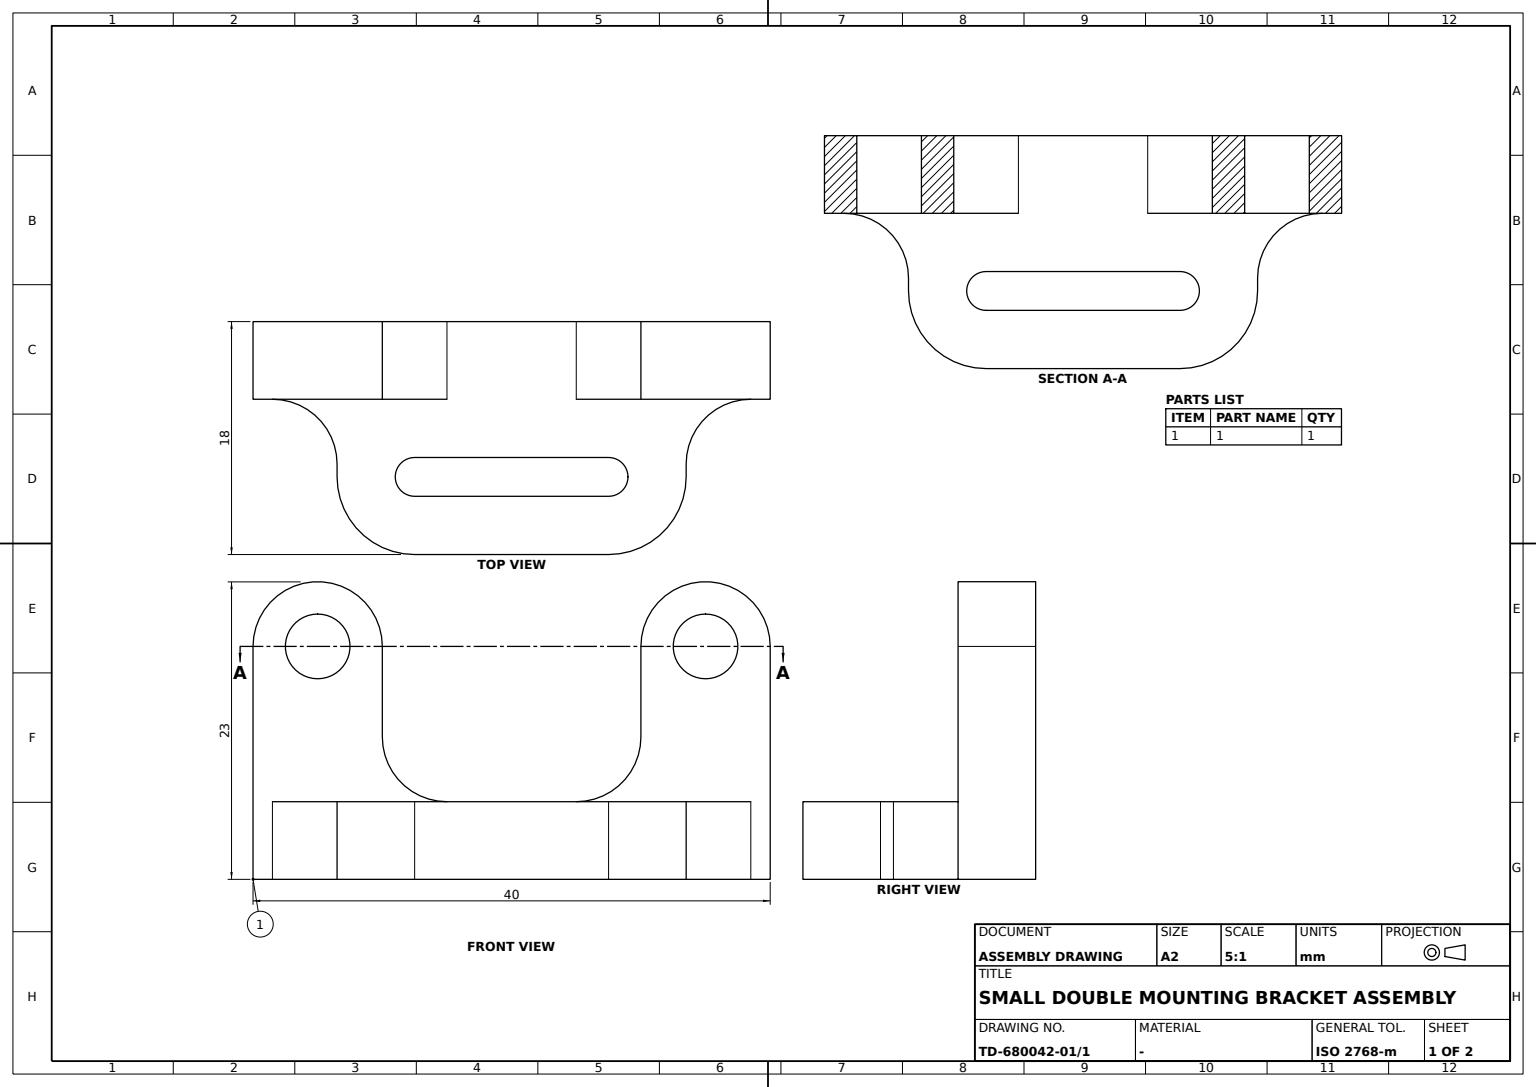
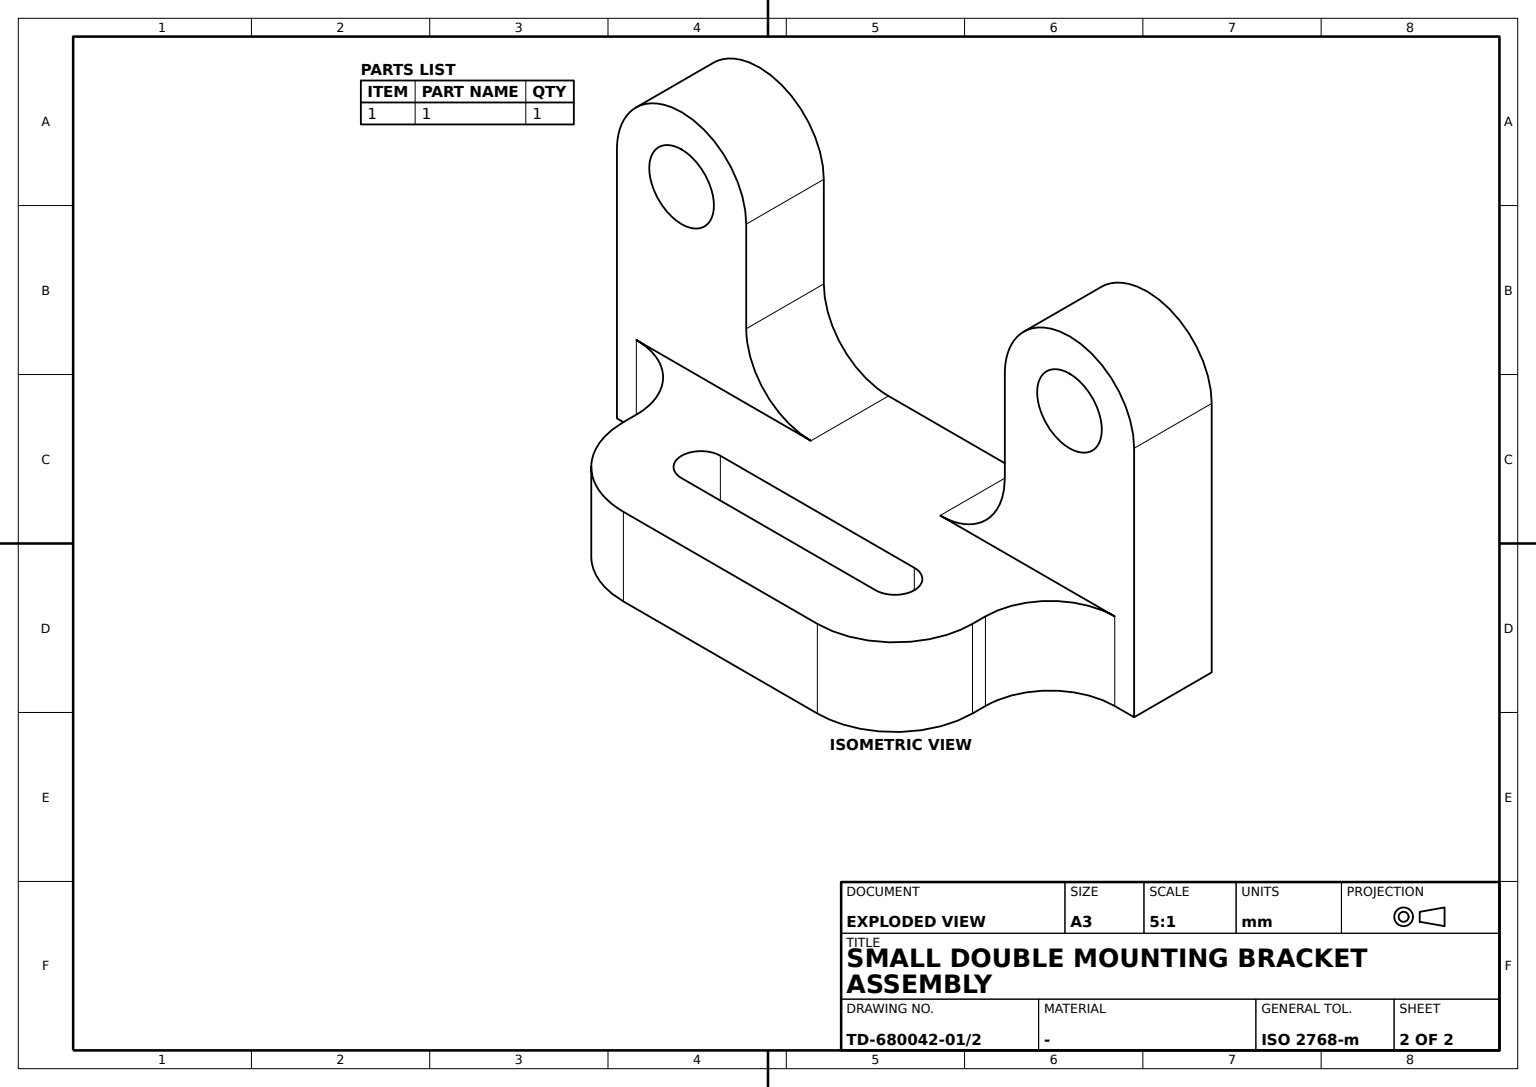
ISO-10303-21;
HEADER;
FILE_DESCRIPTION((''),'2;1');
FILE_NAME('','',(''),(''),'','','');
FILE_SCHEMA(('AUTOMOTIVE_DESIGN'));
ENDSEC;
DATA;
#1=APPLICATION_CONTEXT('');
#2=PRODUCT_CONTEXT('',#1,'mechanical');
#3=PRODUCT('','','',(#2));
#4=PRODUCT_DEFINITION_FORMATION('','',#3);
#5=PRODUCT_DEFINITION_CONTEXT('',#1,'design');
#6=PRODUCT_DEFINITION('','',#4,#5);
#7=PRODUCT_DEFINITION_SHAPE('','',#6);
#8=(LENGTH_UNIT()NAMED_UNIT(*)SI_UNIT(.MILLI.,.METRE.));
#9=(NAMED_UNIT(*)PLANE_ANGLE_UNIT()SI_UNIT($,.RADIAN.));
#10=(NAMED_UNIT(*)SI_UNIT($,.STERADIAN.)SOLID_ANGLE_UNIT());
#11=UNCERTAINTY_MEASURE_WITH_UNIT(LENGTH_MEASURE(1.E-05),#8,'distance_accuracy_value','');
#12=(GEOMETRIC_REPRESENTATION_CONTEXT(3)GLOBAL_UNCERTAINTY_ASSIGNED_CONTEXT((#11))GLOBAL_UNIT_ASSIGNED_CONTEXT((#8,#9,#10))REPRESENTATION_CONTEXT('',''));
#13=CARTESIAN_POINT('',(-5.,-6.,6.));
#14=VERTEX_POINT('',#13);
#15=CARTESIAN_POINT('',(-10.,-6.,11.));
#16=VERTEX_POINT('',#15);
#17=CARTESIAN_POINT('',(-5.,-6.,11.));
#18=DIRECTION('',(0.,1.,0.));
#19=DIRECTION('',(0.,0.,1.));
#20=AXIS2_PLACEMENT_3D('',#17,#18,#19);
#21=CIRCLE('',#20,5.);
#22=EDGE_CURVE('',#14,#16,#21,.T.);
#23=ORIENTED_EDGE('',*,*,#22,.T.);
#24=CARTESIAN_POINT('',(-10.,-6.,18.));
#25=VERTEX_POINT('',#24);
#26=DIRECTION('',(0.,0.,-1.));
#27=VECTOR('',#26,1000.);
#28=LINE('',#24,#27);
#29=EDGE_CURVE('',#25,#16,#28,.T.);
#30=ORIENTED_EDGE('',*,*,#29,.F.);
#31=CARTESIAN_POINT('',(-20.,-6.,18.));
#32=VERTEX_POINT('',#31);
#33=CARTESIAN_POINT('',(-15.,-6.,18.));
#34=DIRECTION('',(0.,-1.,0.));
#35=DIRECTION('',(1.,0.,0.));
#36=AXIS2_PLACEMENT_3D('',#33,#34,#35);
#37=CIRCLE('',#36,5.);
#38=EDGE_CURVE('',#25,#32,#37,.T.);
#39=ORIENTED_EDGE('',*,*,#38,.T.);
#40=CARTESIAN_POINT('',(-20.,-6.,0.));
#41=VERTEX_POINT('',#40);
#42=LINE('',#31,#27);
#43=EDGE_CURVE('',#32,#41,#42,.T.);
#44=ORIENTED_EDGE('',*,*,#43,.T.);
#45=CARTESIAN_POINT('',(-18.5,-6.,0.));
#46=VERTEX_POINT('',#45);
#47=CARTESIAN_POINT('',(-13.5,-6.,0.));
#48=DIRECTION('',(-1.,0.,0.));
#49=VECTOR('',#48,1000.);
#50=LINE('',#47,#49);
#51=EDGE_CURVE('',#46,#41,#50,.T.);
#52=ORIENTED_EDGE('',*,*,#51,.F.);
#53=CARTESIAN_POINT('',(-18.5,-6.,6.));
#54=VERTEX_POINT('',#53);
#55=VECTOR('',#19,1000.);
#56=LINE('',#53,#55);
#57=EDGE_CURVE('',#46,#54,#56,.T.);
#58=ORIENTED_EDGE('',*,*,#57,.T.);
#59=CARTESIAN_POINT('',(20.,-6.,6.));
#60=LINE('',#59,#49);
#61=EDGE_CURVE('',#14,#54,#60,.T.);
#62=ORIENTED_EDGE('',*,*,#61,.F.);
#63=EDGE_LOOP('',(#23,#30,#39,#44,#52,#58,#62));
#64=FACE_OUTER_BOUND('',#63,.T.);
#65=CARTESIAN_POINT('',(-15.,-6.,20.5));
#66=VERTEX_POINT('',#65);
#67=CARTESIAN_POINT('',(-15.,-6.,15.5));
#68=VERTEX_POINT('',#67);
#69=CIRCLE('',#36,2.5);
#70=EDGE_CURVE('',#66,#68,#69,.T.);
#71=ORIENTED_EDGE('',*,*,#70,.F.);
#72=EDGE_CURVE('',#68,#66,#69,.T.);
#73=ORIENTED_EDGE('',*,*,#72,.F.);
#74=EDGE_LOOP('',(#71,#73));
#75=FACE_BOUND('',#74,.T.);
#76=CARTESIAN_POINT('',(20.,-6.,18.));
#77=AXIS2_PLACEMENT_3D('',#76,#18,#19);
#78=PLANE('',#77);
#79=ADVANCED_FACE('',(#64,#75),#78,.F.);
#80=CARTESIAN_POINT('',(-13.5,-11.,6.));
#81=VERTEX_POINT('',#80);
#82=CARTESIAN_POINT('',(-18.5,-11.,6.));
#83=AXIS2_PLACEMENT_3D('',#82,#26,#48);
#84=CIRCLE('',#83,5.);
#85=EDGE_CURVE('',#54,#81,#84,.T.);
#86=ORIENTED_EDGE('',*,*,#85,.F.);
#87=ORIENTED_EDGE('',*,*,#57,.F.);
#88=CARTESIAN_POINT('',(-13.5,-11.,0.));
#89=VERTEX_POINT('',#88);
#90=CARTESIAN_POINT('',(-18.5,-11.,0.));
#91=AXIS2_PLACEMENT_3D('',#90,#19,#34);
#92=CIRCLE('',#91,5.);
#93=EDGE_CURVE('',#89,#46,#92,.T.);
#94=ORIENTED_EDGE('',*,*,#93,.F.);
#95=LINE('',#88,#27);
#96=EDGE_CURVE('',#81,#89,#95,.T.);
#97=ORIENTED_EDGE('',*,*,#96,.F.);
#98=EDGE_LOOP('',(#86,#87,#94,#97));
#99=FACE_OUTER_BOUND('',#98,.T.);
#100=CARTESIAN_POINT('',(-18.5,-11.,18.));
#101=AXIS2_PLACEMENT_3D('',#100,#26,#18);
#102=CYLINDRICAL_SURFACE('',#101,5.);
#103=ADVANCED_FACE('',(#99),#102,.F.);
#104=CARTESIAN_POINT('',(9.,-12.,0.));
#105=VERTEX_POINT('',#104);
#106=CARTESIAN_POINT('',(9.,-12.,6.));
#107=VERTEX_POINT('',#106);
#108=LINE('',#104,#55);
#109=EDGE_CURVE('',#105,#107,#108,.T.);
#110=ORIENTED_EDGE('',*,*,#109,.F.);
#111=CARTESIAN_POINT('',(7.5,-13.5,0.));
#112=VERTEX_POINT('',#111);
#113=CARTESIAN_POINT('',(7.5,-12.,0.));
#114=AXIS2_PLACEMENT_3D('',#113,#19,#35);
#115=CIRCLE('',#114,1.5);
#116=EDGE_CURVE('',#112,#105,#115,.T.);
#117=ORIENTED_EDGE('',*,*,#116,.F.);
#118=CARTESIAN_POINT('',(7.5,-13.5,6.));
#119=VERTEX_POINT('',#118);
#120=LINE('',#111,#27);
#121=EDGE_CURVE('',#119,#112,#120,.T.);
#122=ORIENTED_EDGE('',*,*,#121,.F.);
#123=CARTESIAN_POINT('',(7.5,-12.,6.));
#124=AXIS2_PLACEMENT_3D('',#123,#19,#35);
#125=CIRCLE('',#124,1.5);
#126=EDGE_CURVE('',#119,#107,#125,.T.);
#127=ORIENTED_EDGE('',*,*,#126,.T.);
#128=EDGE_LOOP('',(#110,#117,#122,#127));
#129=FACE_OUTER_BOUND('',#128,.T.);
#130=CYLINDRICAL_SURFACE('',#114,1.5);
#131=ADVANCED_FACE('',(#129),#130,.F.);
#132=CARTESIAN_POINT('',(10.,-6.,11.));
#133=VERTEX_POINT('',#132);
#134=CARTESIAN_POINT('',(5.,-6.,6.));
#135=VERTEX_POINT('',#134);
#136=CARTESIAN_POINT('',(5.,-6.,11.));
#137=AXIS2_PLACEMENT_3D('',#136,#18,#19);
#138=CIRCLE('',#137,5.);
#139=EDGE_CURVE('',#133,#135,#138,.T.);
#140=ORIENTED_EDGE('',*,*,#139,.F.);
#141=CARTESIAN_POINT('',(10.,0.,11.));
#142=VERTEX_POINT('',#141);
#143=VECTOR('',#34,1000.);
#144=LINE('',#132,#143);
#145=EDGE_CURVE('',#142,#133,#144,.T.);
#146=ORIENTED_EDGE('',*,*,#145,.F.);
#147=CARTESIAN_POINT('',(5.,0.,6.));
#148=VERTEX_POINT('',#147);
#149=CARTESIAN_POINT('',(5.,0.,11.));
#150=AXIS2_PLACEMENT_3D('',#149,#34,#26);
#151=CIRCLE('',#150,5.);
#152=EDGE_CURVE('',#148,#142,#151,.T.);
#153=ORIENTED_EDGE('',*,*,#152,.F.);
#154=VECTOR('',#18,1000.);
#155=LINE('',#147,#154);
#156=EDGE_CURVE('',#135,#148,#155,.T.);
#157=ORIENTED_EDGE('',*,*,#156,.F.);
#158=EDGE_LOOP('',(#140,#146,#153,#157));
#159=FACE_OUTER_BOUND('',#158,.T.);
#160=CARTESIAN_POINT('',(5.,34.,11.));
#161=AXIS2_PLACEMENT_3D('',#160,#18,#19);
#162=CYLINDRICAL_SURFACE('',#161,5.);
#163=ADVANCED_FACE('',(#159),#162,.F.);
#164=CARTESIAN_POINT('',(-7.5,-10.5,6.));
#165=VERTEX_POINT('',#164);
#166=CARTESIAN_POINT('',(-7.5,-13.5,6.));
#167=VERTEX_POINT('',#166);
#168=CARTESIAN_POINT('',(-7.5,-12.,6.));
#169=AXIS2_PLACEMENT_3D('',#168,#19,#35);
#170=CIRCLE('',#169,1.5);
#171=EDGE_CURVE('',#165,#167,#170,.T.);
#172=ORIENTED_EDGE('',*,*,#171,.T.);
#173=CARTESIAN_POINT('',(-7.5,-13.5,0.));
#174=VERTEX_POINT('',#173);
#175=LINE('',#173,#27);
#176=EDGE_CURVE('',#167,#174,#175,.T.);
#177=ORIENTED_EDGE('',*,*,#176,.T.);
#178=CARTESIAN_POINT('',(-7.5,-10.5,0.));
#179=VERTEX_POINT('',#178);
#180=CARTESIAN_POINT('',(-7.5,-12.,0.));
#181=AXIS2_PLACEMENT_3D('',#180,#19,#35);
#182=CIRCLE('',#181,1.5);
#183=EDGE_CURVE('',#179,#174,#182,.T.);
#184=ORIENTED_EDGE('',*,*,#183,.F.);
#185=LINE('',#178,#27);
#186=EDGE_CURVE('',#165,#179,#185,.T.);
#187=ORIENTED_EDGE('',*,*,#186,.F.);
#188=EDGE_LOOP('',(#172,#177,#184,#187));
#189=FACE_OUTER_BOUND('',#188,.T.);
#190=CYLINDRICAL_SURFACE('',#181,1.5);
#191=ADVANCED_FACE('',(#189),#190,.F.);
#192=CARTESIAN_POINT('',(13.5,-11.,6.));
#193=VERTEX_POINT('',#192);
#194=CARTESIAN_POINT('',(13.5,-12.,6.));
#195=VERTEX_POINT('',#194);
#196=CARTESIAN_POINT('',(13.5,-6.,6.));
#197=LINE('',#196,#143);
#198=EDGE_CURVE('',#193,#195,#197,.T.);
#199=ORIENTED_EDGE('',*,*,#198,.T.);
#200=CARTESIAN_POINT('',(13.5,-12.,0.));
#201=VERTEX_POINT('',#200);
#202=LINE('',#200,#27);
#203=EDGE_CURVE('',#195,#201,#202,.T.);
#204=ORIENTED_EDGE('',*,*,#203,.T.);
#205=CARTESIAN_POINT('',(13.5,-11.,0.));
#206=VERTEX_POINT('',#205);
#207=CARTESIAN_POINT('',(13.5,-6.,0.));
#208=LINE('',#207,#143);
#209=EDGE_CURVE('',#206,#201,#208,.T.);
#210=ORIENTED_EDGE('',*,*,#209,.F.);
#211=LINE('',#192,#55);
#212=EDGE_CURVE('',#206,#193,#211,.T.);
#213=ORIENTED_EDGE('',*,*,#212,.T.);
#214=EDGE_LOOP('',(#199,#204,#210,#213));
#215=FACE_OUTER_BOUND('',#214,.T.);
#216=AXIS2_PLACEMENT_3D('',#207,#48,#34);
#217=PLANE('',#216);
#218=ADVANCED_FACE('',(#215),#217,.F.);
#219=CARTESIAN_POINT('',(-20.,0.,18.));
#220=VERTEX_POINT('',#219);
#221=LINE('',#219,#143);
#222=EDGE_CURVE('',#220,#32,#221,.T.);
#223=ORIENTED_EDGE('',*,*,#222,.T.);
#224=ORIENTED_EDGE('',*,*,#38,.F.);
#225=CARTESIAN_POINT('',(-10.,0.,18.));
#226=VERTEX_POINT('',#225);
#227=CARTESIAN_POINT('',(-10.,34.,18.));
#228=LINE('',#227,#143);
#229=EDGE_CURVE('',#226,#25,#228,.T.);
#230=ORIENTED_EDGE('',*,*,#229,.F.);
#231=CARTESIAN_POINT('',(-15.,0.,18.));
#232=AXIS2_PLACEMENT_3D('',#231,#34,#35);
#233=CIRCLE('',#232,5.);
#234=EDGE_CURVE('',#226,#220,#233,.T.);
#235=ORIENTED_EDGE('',*,*,#234,.T.);
#236=EDGE_LOOP('',(#223,#224,#230,#235));
#237=FACE_OUTER_BOUND('',#236,.T.);
#238=AXIS2_PLACEMENT_3D('',#231,#34,#26);
#239=CYLINDRICAL_SURFACE('',#238,5.);
#240=ADVANCED_FACE('',(#237),#239,.T.);
#241=CARTESIAN_POINT('',(15.,0.,15.5));
#242=VERTEX_POINT('',#241);
#243=CARTESIAN_POINT('',(15.,0.,20.5));
#244=VERTEX_POINT('',#243);
#245=CARTESIAN_POINT('',(15.,0.,18.));
#246=AXIS2_PLACEMENT_3D('',#245,#34,#35);
#247=CIRCLE('',#246,2.5);
#248=EDGE_CURVE('',#242,#244,#247,.T.);
#249=ORIENTED_EDGE('',*,*,#248,.T.);
#250=EDGE_CURVE('',#244,#242,#247,.T.);
#251=ORIENTED_EDGE('',*,*,#250,.T.);
#252=EDGE_LOOP('',(#249,#251));
#253=FACE_BOUND('',#252,.T.);
#254=CARTESIAN_POINT('',(-15.,0.,15.5));
#255=VERTEX_POINT('',#254);
#256=CARTESIAN_POINT('',(-15.,0.,20.5));
#257=VERTEX_POINT('',#256);
#258=CIRCLE('',#232,2.5);
#259=EDGE_CURVE('',#255,#257,#258,.T.);
#260=ORIENTED_EDGE('',*,*,#259,.T.);
#261=EDGE_CURVE('',#257,#255,#258,.T.);
#262=ORIENTED_EDGE('',*,*,#261,.T.);
#263=EDGE_LOOP('',(#260,#262));
#264=FACE_BOUND('',#263,.T.);
#265=CARTESIAN_POINT('',(-10.,0.,11.));
#266=VERTEX_POINT('',#265);
#267=CARTESIAN_POINT('',(-10.,0.,0.));
#268=LINE('',#267,#27);
#269=EDGE_CURVE('',#226,#266,#268,.T.);
#270=ORIENTED_EDGE('',*,*,#269,.T.);
#271=CARTESIAN_POINT('',(-5.,0.,6.));
#272=VERTEX_POINT('',#271);
#273=CARTESIAN_POINT('',(-5.,0.,11.));
#274=AXIS2_PLACEMENT_3D('',#273,#34,#26);
#275=CIRCLE('',#274,5.);
#276=EDGE_CURVE('',#266,#272,#275,.T.);
#277=ORIENTED_EDGE('',*,*,#276,.T.);
#278=CARTESIAN_POINT('',(20.,0.,6.));
#279=VECTOR('',#35,1000.);
#280=LINE('',#278,#279);
#281=EDGE_CURVE('',#272,#148,#280,.T.);
#282=ORIENTED_EDGE('',*,*,#281,.T.);
#283=ORIENTED_EDGE('',*,*,#152,.T.);
#284=CARTESIAN_POINT('',(10.,0.,18.));
#285=VERTEX_POINT('',#284);
#286=CARTESIAN_POINT('',(10.,0.,0.));
#287=LINE('',#286,#55);
#288=EDGE_CURVE('',#142,#285,#287,.T.);
#289=ORIENTED_EDGE('',*,*,#288,.T.);
#290=CARTESIAN_POINT('',(20.,0.,18.));
#291=VERTEX_POINT('',#290);
#292=CIRCLE('',#246,5.);
#293=EDGE_CURVE('',#291,#285,#292,.T.);
#294=ORIENTED_EDGE('',*,*,#293,.F.);
#295=CARTESIAN_POINT('',(20.,0.,0.));
#296=VERTEX_POINT('',#295);
#297=LINE('',#295,#55);
#298=EDGE_CURVE('',#296,#291,#297,.T.);
#299=ORIENTED_EDGE('',*,*,#298,.F.);
#300=CARTESIAN_POINT('',(-20.,0.,0.));
#301=VERTEX_POINT('',#300);
#302=LINE('',#295,#49);
#303=EDGE_CURVE('',#296,#301,#302,.T.);
#304=ORIENTED_EDGE('',*,*,#303,.T.);
#305=LINE('',#300,#55);
#306=EDGE_CURVE('',#301,#220,#305,.T.);
#307=ORIENTED_EDGE('',*,*,#306,.T.);
#308=ORIENTED_EDGE('',*,*,#234,.F.);
#309=EDGE_LOOP('',(#270,#277,#282,#283,#289,#294,#299,#304,#307,#308));
#310=FACE_OUTER_BOUND('',#309,.T.);
#311=AXIS2_PLACEMENT_3D('',#295,#34,#26);
#312=PLANE('',#311);
#313=ADVANCED_FACE('',(#253,#264,#310),#312,.F.);
#314=LINE('',#256,#143);
#315=EDGE_CURVE('',#257,#66,#314,.T.);
#316=ORIENTED_EDGE('',*,*,#315,.F.);
#317=ORIENTED_EDGE('',*,*,#259,.F.);
#318=LINE('',#254,#143);
#319=EDGE_CURVE('',#255,#68,#318,.T.);
#320=ORIENTED_EDGE('',*,*,#319,.T.);
#321=ORIENTED_EDGE('',*,*,#72,.T.);
#322=EDGE_LOOP('',(#316,#317,#320,#321));
#323=FACE_OUTER_BOUND('',#322,.T.);
#324=CYLINDRICAL_SURFACE('',#238,2.5);
#325=ADVANCED_FACE('',(#323),#324,.F.);
#326=ORIENTED_EDGE('',*,*,#29,.T.);
#327=LINE('',#265,#154);
#328=EDGE_CURVE('',#16,#266,#327,.T.);
#329=ORIENTED_EDGE('',*,*,#328,.T.);
#330=ORIENTED_EDGE('',*,*,#269,.F.);
#331=ORIENTED_EDGE('',*,*,#229,.T.);
#332=EDGE_LOOP('',(#326,#329,#330,#331));
#333=FACE_OUTER_BOUND('',#332,.T.);
#334=AXIS2_PLACEMENT_3D('',#227,#48,#19);
#335=PLANE('',#334);
#336=ADVANCED_FACE('',(#333),#335,.F.);
#337=CARTESIAN_POINT('',(-13.5,-12.,0.));
#338=VERTEX_POINT('',#337);
#339=CARTESIAN_POINT('',(-13.5,-12.,6.));
#340=VERTEX_POINT('',#339);
#341=LINE('',#337,#55);
#342=EDGE_CURVE('',#338,#340,#341,.T.);
#343=ORIENTED_EDGE('',*,*,#342,.F.);
#344=CARTESIAN_POINT('',(-7.5,-18.,0.));
#345=VERTEX_POINT('',#344);
#346=AXIS2_PLACEMENT_3D('',#180,#26,#34);
#347=CIRCLE('',#346,6.);
#348=EDGE_CURVE('',#345,#338,#347,.T.);
#349=ORIENTED_EDGE('',*,*,#348,.F.);
#350=CARTESIAN_POINT('',(-7.5,-18.,6.));
#351=VERTEX_POINT('',#350);
#352=LINE('',#350,#27);
#353=EDGE_CURVE('',#351,#345,#352,.T.);
#354=ORIENTED_EDGE('',*,*,#353,.F.);
#355=AXIS2_PLACEMENT_3D('',#168,#19,#48);
#356=CIRCLE('',#355,6.);
#357=EDGE_CURVE('',#340,#351,#356,.T.);
#358=ORIENTED_EDGE('',*,*,#357,.F.);
#359=EDGE_LOOP('',(#343,#349,#354,#358));
#360=FACE_OUTER_BOUND('',#359,.T.);
#361=AXIS2_PLACEMENT_3D('',#180,#19,#34);
#362=CYLINDRICAL_SURFACE('',#361,6.);
#363=ADVANCED_FACE('',(#360),#362,.T.);
#364=CARTESIAN_POINT('',(7.5,-18.,6.));
#365=VERTEX_POINT('',#364);
#366=AXIS2_PLACEMENT_3D('',#123,#19,#48);
#367=CIRCLE('',#366,6.);
#368=EDGE_CURVE('',#365,#195,#367,.T.);
#369=ORIENTED_EDGE('',*,*,#368,.F.);
#370=CARTESIAN_POINT('',(7.5,-18.,0.));
#371=VERTEX_POINT('',#370);
#372=LINE('',#364,#55);
#373=EDGE_CURVE('',#371,#365,#372,.T.);
#374=ORIENTED_EDGE('',*,*,#373,.F.);
#375=AXIS2_PLACEMENT_3D('',#113,#26,#34);
#376=CIRCLE('',#375,6.);
#377=EDGE_CURVE('',#201,#371,#376,.T.);
#378=ORIENTED_EDGE('',*,*,#377,.F.);
#379=ORIENTED_EDGE('',*,*,#203,.F.);
#380=EDGE_LOOP('',(#369,#374,#378,#379));
#381=FACE_OUTER_BOUND('',#380,.T.);
#382=AXIS2_PLACEMENT_3D('',#123,#19,#34);
#383=CYLINDRICAL_SURFACE('',#382,6.);
#384=ADVANCED_FACE('',(#381),#383,.T.);
#385=CARTESIAN_POINT('',(20.,-18.,0.));
#386=LINE('',#385,#49);
#387=EDGE_CURVE('',#371,#345,#386,.T.);
#388=ORIENTED_EDGE('',*,*,#387,.F.);
#389=ORIENTED_EDGE('',*,*,#373,.T.);
#390=CARTESIAN_POINT('',(20.,-18.,6.));
#391=LINE('',#390,#49);
#392=EDGE_CURVE('',#365,#351,#391,.T.);
#393=ORIENTED_EDGE('',*,*,#392,.T.);
#394=ORIENTED_EDGE('',*,*,#353,.T.);
#395=EDGE_LOOP('',(#388,#389,#393,#394));
#396=FACE_OUTER_BOUND('',#395,.T.);
#397=AXIS2_PLACEMENT_3D('',#390,#18,#19);
#398=PLANE('',#397);
#399=ADVANCED_FACE('',(#396),#398,.F.);
#400=ORIENTED_EDGE('',*,*,#293,.T.);
#401=CARTESIAN_POINT('',(10.,-6.,18.));
#402=VERTEX_POINT('',#401);
#403=CARTESIAN_POINT('',(10.,34.,18.));
#404=LINE('',#403,#143);
#405=EDGE_CURVE('',#285,#402,#404,.T.);
#406=ORIENTED_EDGE('',*,*,#405,.T.);
#407=VERTEX_POINT('',#76);
#408=CARTESIAN_POINT('',(15.,-6.,18.));
#409=AXIS2_PLACEMENT_3D('',#408,#34,#35);
#410=CIRCLE('',#409,5.);
#411=EDGE_CURVE('',#407,#402,#410,.T.);
#412=ORIENTED_EDGE('',*,*,#411,.F.);
#413=LINE('',#290,#143);
#414=EDGE_CURVE('',#291,#407,#413,.T.);
#415=ORIENTED_EDGE('',*,*,#414,.F.);
#416=EDGE_LOOP('',(#400,#406,#412,#415));
#417=FACE_OUTER_BOUND('',#416,.T.);
#418=AXIS2_PLACEMENT_3D('',#245,#34,#26);
#419=CYLINDRICAL_SURFACE('',#418,5.);
#420=ADVANCED_FACE('',(#417),#419,.T.);
#421=CARTESIAN_POINT('',(20.,-6.,0.));
#422=VERTEX_POINT('',#421);
#423=LINE('',#385,#154);
#424=EDGE_CURVE('',#422,#296,#423,.T.);
#425=ORIENTED_EDGE('',*,*,#424,.T.);
#426=ORIENTED_EDGE('',*,*,#298,.T.);
#427=ORIENTED_EDGE('',*,*,#414,.T.);
#428=LINE('',#76,#27);
#429=EDGE_CURVE('',#407,#422,#428,.T.);
#430=ORIENTED_EDGE('',*,*,#429,.T.);
#431=EDGE_LOOP('',(#425,#426,#427,#430));
#432=FACE_OUTER_BOUND('',#431,.T.);
#433=AXIS2_PLACEMENT_3D('',#295,#35,#26);
#434=PLANE('',#433);
#435=ADVANCED_FACE('',(#432),#434,.T.);
#436=CARTESIAN_POINT('',(15.,-6.,15.5));
#437=VERTEX_POINT('',#436);
#438=CARTESIAN_POINT('',(15.,-6.,20.5));
#439=VERTEX_POINT('',#438);
#440=CIRCLE('',#409,2.5);
#441=EDGE_CURVE('',#437,#439,#440,.T.);
#442=ORIENTED_EDGE('',*,*,#441,.F.);
#443=EDGE_CURVE('',#439,#437,#440,.T.);
#444=ORIENTED_EDGE('',*,*,#443,.F.);
#445=EDGE_LOOP('',(#442,#444));
#446=FACE_BOUND('',#445,.T.);
#447=CARTESIAN_POINT('',(18.5,-6.,0.));
#448=VERTEX_POINT('',#447);
#449=LINE('',#421,#49);
#450=EDGE_CURVE('',#422,#448,#449,.T.);
#451=ORIENTED_EDGE('',*,*,#450,.F.);
#452=ORIENTED_EDGE('',*,*,#429,.F.);
#453=ORIENTED_EDGE('',*,*,#411,.T.);
#454=CARTESIAN_POINT('',(10.,-6.,6.));
#455=LINE('',#454,#55);
#456=EDGE_CURVE('',#133,#402,#455,.T.);
#457=ORIENTED_EDGE('',*,*,#456,.F.);
#458=ORIENTED_EDGE('',*,*,#139,.T.);
#459=CARTESIAN_POINT('',(18.5,-6.,6.));
#460=VERTEX_POINT('',#459);
#461=EDGE_CURVE('',#460,#135,#60,.T.);
#462=ORIENTED_EDGE('',*,*,#461,.F.);
#463=LINE('',#447,#27);
#464=EDGE_CURVE('',#460,#448,#463,.T.);
#465=ORIENTED_EDGE('',*,*,#464,.T.);
#466=EDGE_LOOP('',(#451,#452,#453,#457,#458,#462,#465));
#467=FACE_OUTER_BOUND('',#466,.T.);
#468=ADVANCED_FACE('',(#446,#467),#78,.F.);
#469=ORIENTED_EDGE('',*,*,#276,.F.);
#470=ORIENTED_EDGE('',*,*,#328,.F.);
#471=ORIENTED_EDGE('',*,*,#22,.F.);
#472=LINE('',#13,#143);
#473=EDGE_CURVE('',#272,#14,#472,.T.);
#474=ORIENTED_EDGE('',*,*,#473,.F.);
#475=EDGE_LOOP('',(#469,#470,#471,#474));
#476=FACE_OUTER_BOUND('',#475,.T.);
#477=CYLINDRICAL_SURFACE('',#20,5.);
#478=ADVANCED_FACE('',(#476),#477,.F.);
#479=ORIENTED_EDGE('',*,*,#121,.T.);
#480=LINE('',#173,#279);
#481=EDGE_CURVE('',#174,#112,#480,.T.);
#482=ORIENTED_EDGE('',*,*,#481,.F.);
#483=ORIENTED_EDGE('',*,*,#176,.F.);
#484=LINE('',#166,#279);
#485=EDGE_CURVE('',#167,#119,#484,.T.);
#486=ORIENTED_EDGE('',*,*,#485,.T.);
#487=EDGE_LOOP('',(#479,#482,#483,#486));
#488=FACE_OUTER_BOUND('',#487,.T.);
#489=AXIS2_PLACEMENT_3D('',#173,#34,#26);
#490=PLANE('',#489);
#491=ADVANCED_FACE('',(#488),#490,.F.);
#492=LINE('',#241,#143);
#493=EDGE_CURVE('',#242,#437,#492,.T.);
#494=ORIENTED_EDGE('',*,*,#493,.T.);
#495=ORIENTED_EDGE('',*,*,#441,.T.);
#496=LINE('',#243,#143);
#497=EDGE_CURVE('',#244,#439,#496,.T.);
#498=ORIENTED_EDGE('',*,*,#497,.F.);
#499=ORIENTED_EDGE('',*,*,#248,.F.);
#500=EDGE_LOOP('',(#494,#495,#498,#499));
#501=FACE_OUTER_BOUND('',#500,.T.);
#502=CYLINDRICAL_SURFACE('',#418,2.5);
#503=ADVANCED_FACE('',(#501),#502,.F.);
#504=ORIENTED_EDGE('',*,*,#222,.F.);
#505=ORIENTED_EDGE('',*,*,#306,.F.);
#506=CARTESIAN_POINT('',(-20.,-18.,0.));
#507=LINE('',#506,#154);
#508=EDGE_CURVE('',#41,#301,#507,.T.);
#509=ORIENTED_EDGE('',*,*,#508,.F.);
#510=ORIENTED_EDGE('',*,*,#43,.F.);
#511=EDGE_LOOP('',(#504,#505,#509,#510));
#512=FACE_OUTER_BOUND('',#511,.T.);
#513=AXIS2_PLACEMENT_3D('',#300,#35,#26);
#514=PLANE('',#513);
#515=ADVANCED_FACE('',(#512),#514,.F.);
#516=ORIENTED_EDGE('',*,*,#96,.T.);
#517=CARTESIAN_POINT('',(-13.5,-18.,0.));
#518=LINE('',#517,#154);
#519=EDGE_CURVE('',#338,#89,#518,.T.);
#520=ORIENTED_EDGE('',*,*,#519,.F.);
#521=ORIENTED_EDGE('',*,*,#342,.T.);
#522=CARTESIAN_POINT('',(-13.5,-18.,6.));
#523=LINE('',#522,#154);
#524=EDGE_CURVE('',#340,#81,#523,.T.);
#525=ORIENTED_EDGE('',*,*,#524,.T.);
#526=EDGE_LOOP('',(#516,#520,#521,#525));
#527=FACE_OUTER_BOUND('',#526,.T.);
#528=AXIS2_PLACEMENT_3D('',#517,#35,#26);
#529=PLANE('',#528);
#530=ADVANCED_FACE('',(#527),#529,.F.);
#531=CARTESIAN_POINT('',(7.5,-10.5,0.));
#532=VERTEX_POINT('',#531);
#533=LINE('',#531,#49);
#534=EDGE_CURVE('',#532,#179,#533,.T.);
#535=ORIENTED_EDGE('',*,*,#534,.F.);
#536=CARTESIAN_POINT('',(7.5,-10.5,6.));
#537=VERTEX_POINT('',#536);
#538=LINE('',#531,#27);
#539=EDGE_CURVE('',#537,#532,#538,.T.);
#540=ORIENTED_EDGE('',*,*,#539,.F.);
#541=LINE('',#536,#49);
#542=EDGE_CURVE('',#537,#165,#541,.T.);
#543=ORIENTED_EDGE('',*,*,#542,.T.);
#544=ORIENTED_EDGE('',*,*,#186,.T.);
#545=EDGE_LOOP('',(#535,#540,#543,#544));
#546=FACE_OUTER_BOUND('',#545,.T.);
#547=AXIS2_PLACEMENT_3D('',#531,#18,#19);
#548=PLANE('',#547);
#549=ADVANCED_FACE('',(#546),#548,.F.);
#550=ORIENTED_EDGE('',*,*,#424,.F.);
#551=ORIENTED_EDGE('',*,*,#450,.T.);
#552=CARTESIAN_POINT('',(18.5,-11.,0.));
#553=AXIS2_PLACEMENT_3D('',#552,#19,#34);
#554=CIRCLE('',#553,5.);
#555=EDGE_CURVE('',#448,#206,#554,.T.);
#556=ORIENTED_EDGE('',*,*,#555,.T.);
#557=ORIENTED_EDGE('',*,*,#209,.T.);
#558=ORIENTED_EDGE('',*,*,#377,.T.);
#559=ORIENTED_EDGE('',*,*,#387,.T.);
#560=ORIENTED_EDGE('',*,*,#348,.T.);
#561=ORIENTED_EDGE('',*,*,#519,.T.);
#562=ORIENTED_EDGE('',*,*,#93,.T.);
#563=ORIENTED_EDGE('',*,*,#51,.T.);
#564=ORIENTED_EDGE('',*,*,#508,.T.);
#565=ORIENTED_EDGE('',*,*,#303,.F.);
#566=EDGE_LOOP('',(#550,#551,#556,#557,#558,#559,#560,#561,#562,#563,#564,#565));
#567=FACE_OUTER_BOUND('',#566,.T.);
#568=EDGE_CURVE('',#105,#532,#115,.T.);
#569=ORIENTED_EDGE('',*,*,#568,.T.);
#570=ORIENTED_EDGE('',*,*,#534,.T.);
#571=ORIENTED_EDGE('',*,*,#183,.T.);
#572=ORIENTED_EDGE('',*,*,#481,.T.);
#573=ORIENTED_EDGE('',*,*,#116,.T.);
#574=EDGE_LOOP('',(#569,#570,#571,#572,#573));
#575=FACE_BOUND('',#574,.T.);
#576=AXIS2_PLACEMENT_3D('',#385,#19,#34);
#577=PLANE('',#576);
#578=ADVANCED_FACE('',(#567,#575),#577,.F.);
#579=ORIENTED_EDGE('',*,*,#456,.T.);
#580=ORIENTED_EDGE('',*,*,#405,.F.);
#581=ORIENTED_EDGE('',*,*,#288,.F.);
#582=ORIENTED_EDGE('',*,*,#145,.T.);
#583=EDGE_LOOP('',(#579,#580,#581,#582));
#584=FACE_OUTER_BOUND('',#583,.T.);
#585=CARTESIAN_POINT('',(10.,34.,6.));
#586=AXIS2_PLACEMENT_3D('',#585,#35,#26);
#587=PLANE('',#586);
#588=ADVANCED_FACE('',(#584),#587,.F.);
#589=ORIENTED_EDGE('',*,*,#70,.T.);
#590=ORIENTED_EDGE('',*,*,#319,.F.);
#591=ORIENTED_EDGE('',*,*,#261,.F.);
#592=ORIENTED_EDGE('',*,*,#315,.T.);
#593=EDGE_LOOP('',(#589,#590,#591,#592));
#594=FACE_OUTER_BOUND('',#593,.T.);
#595=ADVANCED_FACE('',(#594),#324,.F.);
#596=ORIENTED_EDGE('',*,*,#485,.F.);
#597=ORIENTED_EDGE('',*,*,#171,.F.);
#598=ORIENTED_EDGE('',*,*,#542,.F.);
#599=EDGE_CURVE('',#107,#537,#125,.T.);
#600=ORIENTED_EDGE('',*,*,#599,.F.);
#601=ORIENTED_EDGE('',*,*,#126,.F.);
#602=EDGE_LOOP('',(#596,#597,#598,#600,#601));
#603=FACE_BOUND('',#602,.T.);
#604=ORIENTED_EDGE('',*,*,#392,.F.);
#605=ORIENTED_EDGE('',*,*,#368,.T.);
#606=ORIENTED_EDGE('',*,*,#198,.F.);
#607=CARTESIAN_POINT('',(18.5,-11.,6.));
#608=AXIS2_PLACEMENT_3D('',#607,#26,#48);
#609=CIRCLE('',#608,5.);
#610=EDGE_CURVE('',#193,#460,#609,.T.);
#611=ORIENTED_EDGE('',*,*,#610,.T.);
#612=ORIENTED_EDGE('',*,*,#461,.T.);
#613=ORIENTED_EDGE('',*,*,#156,.T.);
#614=ORIENTED_EDGE('',*,*,#281,.F.);
#615=ORIENTED_EDGE('',*,*,#473,.T.);
#616=ORIENTED_EDGE('',*,*,#61,.T.);
#617=ORIENTED_EDGE('',*,*,#85,.T.);
#618=ORIENTED_EDGE('',*,*,#524,.F.);
#619=ORIENTED_EDGE('',*,*,#357,.T.);
#620=EDGE_LOOP('',(#604,#605,#606,#611,#612,#613,#614,#615,#616,#617,#618,#619));
#621=FACE_OUTER_BOUND('',#620,.T.);
#622=AXIS2_PLACEMENT_3D('',#59,#26,#48);
#623=PLANE('',#622);
#624=ADVANCED_FACE('',(#603,#621),#623,.F.);
#625=ORIENTED_EDGE('',*,*,#493,.F.);
#626=ORIENTED_EDGE('',*,*,#250,.F.);
#627=ORIENTED_EDGE('',*,*,#497,.T.);
#628=ORIENTED_EDGE('',*,*,#443,.T.);
#629=EDGE_LOOP('',(#625,#626,#627,#628));
#630=FACE_OUTER_BOUND('',#629,.T.);
#631=ADVANCED_FACE('',(#630),#502,.F.);
#632=ORIENTED_EDGE('',*,*,#568,.F.);
#633=ORIENTED_EDGE('',*,*,#109,.T.);
#634=ORIENTED_EDGE('',*,*,#599,.T.);
#635=ORIENTED_EDGE('',*,*,#539,.T.);
#636=EDGE_LOOP('',(#632,#633,#634,#635));
#637=FACE_OUTER_BOUND('',#636,.T.);
#638=ADVANCED_FACE('',(#637),#130,.F.);
#639=ORIENTED_EDGE('',*,*,#555,.F.);
#640=ORIENTED_EDGE('',*,*,#464,.F.);
#641=ORIENTED_EDGE('',*,*,#610,.F.);
#642=ORIENTED_EDGE('',*,*,#212,.F.);
#643=EDGE_LOOP('',(#639,#640,#641,#642));
#644=FACE_OUTER_BOUND('',#643,.T.);
#645=AXIS2_PLACEMENT_3D('',#552,#26,#18);
#646=CYLINDRICAL_SURFACE('',#645,5.);
#647=ADVANCED_FACE('',(#644),#646,.F.);
#648=CLOSED_SHELL('',(#79,#103,#131,#163,#191,#218,#240,#313,#325,#336,#363,#384,#399,#420,#435,#468,#478,#491,#503,#515,#530,#549,#578,#588,#595,#624,#631,#638,#647));
#649=MANIFOLD_SOLID_BREP('',#648);
#650=ADVANCED_BREP_SHAPE_REPRESENTATION('',(#649),#12);
#651=SHAPE_DEFINITION_REPRESENTATION(#7,#650);
ENDSEC;
END-ISO-10303-21;
